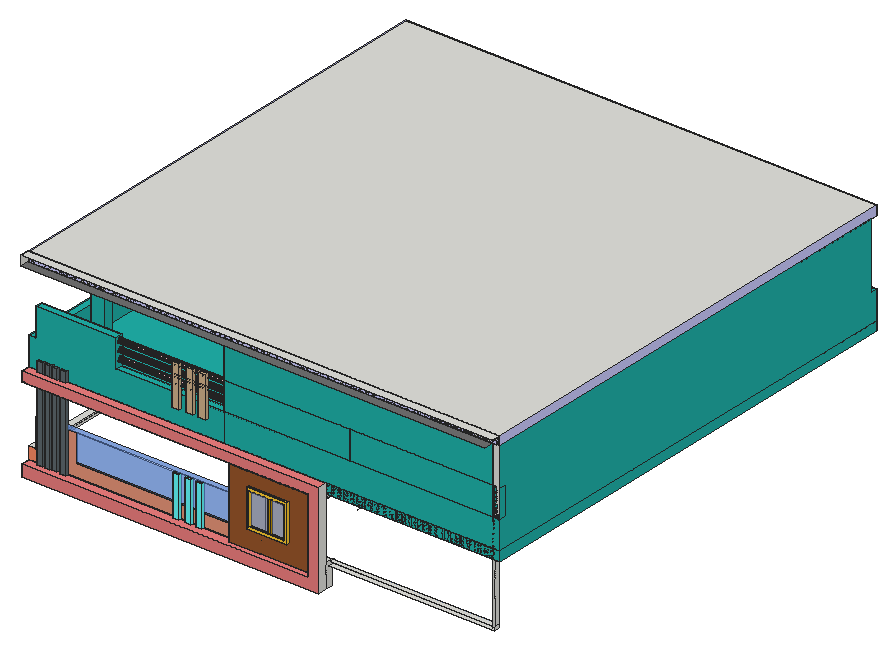
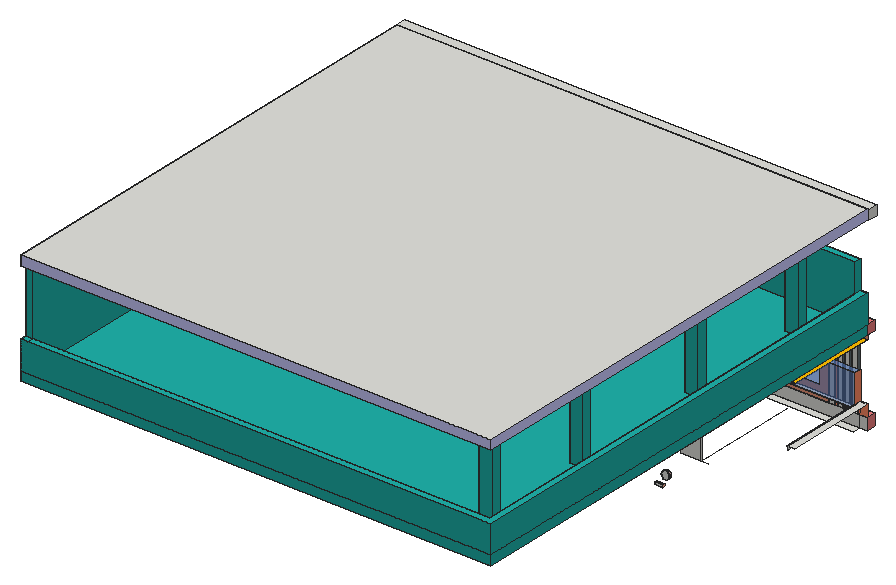
# SketchUp Ruby script. Lengths in inches.
U = 1.inch
M = Sketchup.active_model
def pt(a) = Geom::Point3d.new(a.map { |v| v * U })
def face(e, loops, mat)
  f = e.add_face(loops[0].map { |a| pt(a) })
  loops[1..].each { |l| e.add_face(l.map { |a| pt(a) }).erase! }
  f.material = f.back_material = mat if mat
  f
end
# faces: each face lists its corners as indices into pts; further lists are holes
def faces(e, pts, list, mat = nil) = list.each { |f| face(e, (f[0].is_a?(Array) ? f : [f]).map { |l| l.map { |i| pts[i] } }, mat) }
# xy, xz, yz: faces in a plane at the given z, y or x. An outline is a flat list of corners, or four numbers for a rectangle; further outlines are holes
def ring(l) = l.size == 4 ? [[l[0], l[1]], [l[2], l[1]], [l[2], l[3]], [l[0], l[3]]] : l.each_slice(2).to_a
def flat(e, list, mat, &to3) = list.each { |f| face(e, (f[0].is_a?(Array) ? f : [f]).map { |l| ring(l).map { |u, v| to3.(u, v) } }, mat) }
def xy(e, z, list, mat = nil) = flat(e, list, mat) { |x, y| [x, y, z] }
def xz(e, y, list, mat = nil) = flat(e, list, mat) { |x, z| [x, y, z] }
def yz(e, x, list, mat = nil) = flat(e, list, mat) { |y, z| [x, y, z] }
def lines(e, pts, list) = list.each { |a, b| e.add_line(pt(pts[a]), pt(pts[b])) }
# prism: a flat outline (further loops are holes) pulled along v
def prism(e, loops, v, mat = nil)
  f = face(e, loops, mat); d = Geom::Vector3d.new(v.map { |x| x * U })
  f.pushpull(f.normal.samedirection?(d) ? d.length : -d.length)
end
def box(e, o, s, mat = nil) = prism(e, [[o, [o[0] + s[0], o[1], o[2]], [o[0] + s[0], o[1] + s[1], o[2]], [o[0], o[1] + s[1], o[2]]]], [0, 0, s[2]], mat)
def at(x, y, z, deg = 0) = Geom::Transformation.translation(pt([x, y, z])) * Geom::Transformation.rotation(ORIGIN, Z_AXIS, deg.degrees)
def axes(o, x, y, z) = Geom::Transformation.new([*x, 0, *y, 0, *z, 0, *pt(o).to_a, 1])
def part(name) = M.definitions.add(name)
# library, detail: a bought-in or finely detailed component or shape, given as its bounding box
def library(name, o, s) = part(name).tap { |d| box(d.entities, o, s) }
def detail(e, o, s) = box(e.add_group.entities, o, s)
def put(e, d, t, mat = nil) = e.add_instance(d, t).tap { |i| i.material = mat if mat }
def group(e, t, mat = nil) = e.add_group.tap { |g| g.transformation = t; g.material = mat if mat }.entities
root = M.entities
M.materials.add("[0006_Pink]").color = [255, 192, 203]
M.materials.add("[0013_LightCoral]").color = [240, 128, 128]
M.materials.add("[0014_DarkSalmon]").color = [233, 150, 122]
M.materials.add("[0035_Tan]").color = [210, 180, 140]
M.materials.add("[0082_LightSeaGreen]").color = [32, 178, 170]
M.materials.add("[Color A01]").color = [255, 204, 204]
M.materials.add("[Color B02]").color = [255, 178, 153]
M.materials.add("[Color B03]").color = [255, 140, 101]
M.materials.add("[Color B07]").color = [153, 38, 0]
M.materials.add("[Color D04]").color = [255, 204, 50]
M.materials.add("[Color D05]").color = [255, 191, 0]
M.materials.add("[Color D06]").color = [204, 153, 0]
M.materials.add("[Color H03]").color = [101, 255, 255]
M.materials.add("[Color I01]").color = [204, 204, 255]
M.materials.add("[Color M05]").color = [114, 114, 114]
M.materials.add("[Formica Beige]").color = [211, 187, 149]
M.materials.add("[Formica Speckled Grey]").color = [94, 105, 111]
M.materials.add("[Translucent Glass Blue]").color = [100, 149, 237]
M.materials["[Translucent Glass Blue]"].alpha = 0.5
M.materials.add("[Translucent Glass Sky Reflection]").color = [126, 138, 183]
M.materials["[Translucent Glass Sky Reflection]"].alpha = 0.52
M.materials.add("[Translucent Glass Tinted]").color = [8, 201, 241]
M.materials["[Translucent Glass Tinted]"].alpha = 0.48
M.materials.add("[Wood Cherry Original]").color = [152, 86, 42]
xy(root,251.61,[[1.5625,0,1.5625,12,265.96,12,265.96,6,367.6875,6,367.6875,12,380.39,12,380.39,0],[265.96,6,301.8125,12],[301.8125,6,367.6875,12],[11.0625,12,380.39,21.5]])
xy(root,264.68,[[261.33,6,301.8125,12]])
xy(root,266.86,[[14.35,9,21.23,12],[23.92,9,30.79,12],[32.85,9,39.73,12],[43.48,9,50.35,12],[186.5625,9,194.61,12],
  [202.3125,9,210.36,12],[216.3125,9,224.36,12],[21.23,12,23.92,12.375],[30.79,12,32.85,12.375]])
xy(root,266.86,[[1.5625,0,367,0,367,12,224.36,12,224.36,9,216.3125,9,216.3125,12,210.36,12,210.36,9,202.3125,9,202.3125,12,194.61,12,194.61,9,186.5625,9,186.5625,12,50.35,12,50.35,9,43.48,9,43.48,12,39.73,12,39.73,9,32.85,9,32.85,12,30.79,12,30.79,9,23.92,9,23.92,12,21.23,12,21.23,9,14.35,9,14.35,12,1.5625,12]],"[0013_LightCoral]")
xy(root,267.18,[[301.8125,6,376.3125,12]])
xy(root,273.74,[[23.92,12,30.79,12.375]])
xy(root,275.45,[[61.8125,259.15,72.25,262.15]])
xy(root,277.61,[[10.5625,15.5625,10.6875,20.9375],[10.6875,15.5625,592.5625,20.9375],[10.5625,20.9375,10.6875,21],[10.6875,20.9375,592.5625,21],[10.5625,21,10.6875,127.99]])
xy(root,278.01,[[61.8125,259.15,72.25,262.15]],"[Color B02]")
xy(root,282.11,[[1.5625,12,10.5625,127.99],[10.5625,12,11.0625,127.99],[260.74,12,380.39,21],[380.39,15.5625,592.5625,21],[380.39,21,592.5625,21.5]])
xy(root,291.58,[[286.22,3,337.03,6]],"[Color D04]")
xy(root,294.58,[[311.625,5,315.25,6]])
xy(root,294.58,[[289.22,3,311.625,6],[311.625,3,315.25,5],[315.25,3,334.03,6]],"[Color D04]")
xy(root,294.68,[[181.96,262.15,184.61,265.15],[141.83,265.15,181.96,277.84],[181.96,265.15,184.61,277.84],[184.61,265.15,227.4,277.84]])
xy(root,318.07,[[186.5625,9,194.61,12]],"[Color H03]")
xy(root,318.11,[[21.23,12,32.85,12.375]])
xy(root,318.11,[[202.3125,9,210.36,12],[216.3125,9,224.36,12]],"[Color H03]")
xy(root,318.11,[[10.5625,12,21.23,12,21.23,12.375,32.85,12.375,32.85,12,260.74,12,260.74,21,10.5625,21]],"[Translucent Glass Blue]")
xy(root,324.8,[[49.5,262.15,85.5,265.15],[49.5,265.15,85.5,277.84]])
xy(root,327.74,[[181.96,262.15,184.61,265.15],[141.83,265.15,181.96,277.84],[184.61,265.15,227.4,277.84]])
xy(root,336.15,[[311.625,5,315.25,6]])
xy(root,336.15,[[289.22,3,311.625,6],[311.625,3,315.25,5],[315.25,3,334.03,6]],"[Color D04]")
xy(root,339.15,[[286.22,3,337.03,6]],"[Color D04]")
xy(root,355.61,[[1.5625,12,1.5625,127.99,10.5625,127.99,10.5625,139.1875,381.4375,139.1875,381.4375,12.02,380.39,12]],"[Color D05]")
xy(root,355.8,[[261.33,6,301.8125,12],[301.8125,6,376.3125,12],[10.5625,127.99,36.75,139.1875]])
xy(root,360.74,[[261.33,6,301.8125,12]])
xy(root,360.8,[[1.5625,12,380.39,12,381.4375,12.02,381.4375,139.1875,10.5625,139.1875,10.5625,127.99,1.5625,127.99],[380.39,12,381.4375,12,381.4375,12.02],[381.4375,12,592.5625,12,592.5625,15.5625,419.5,12.66,419.5,12.02,381.4375,12.02],[592.5625,12,601.5625,21.5],[381.4375,12.02,419.5,12.02,419.5,12.66],
  [381.4375,12.02,419.5,12.66,381.4375,12.66],[419.5,12.66,592.5625,15.5625,592.5625,265.15,36.75,265.15,36.75,139.1875,419.5,139.1875],[381.4375,12.66,419.5,139.1875],[592.5625,21.5,601.5625,21.5,601.5625,612,11.0625,612,11.0625,603,592.5625,603],[1.5625,127.99,10.5625,139.1875],
  [1.5625,139.1875,10.5625,265.15],[10.5625,139.1875,36.75,265.15],[1.5625,265.15,11.0625,265.15,11.0625,277.84,10.5625,277.84,10.5625,603,1.5625,603],[11.0625,265.15,592.5625,277.84],[10.5625,277.84,11.0625,603],
  [1.5625,603,11.0625,612]])
xy(root,360.8,[[1.5625,0,367,12]],"[0013_LightCoral]")
xy(root,360.86,[[1.5625,0,367,12]])
xy(root,361.18,[[301.8125,6,376.3125,12]])
xy(root,372.8,[[1.5625,0,380.39,12]],"[0013_LightCoral]")
xy(root,385.3,[[14.35,9,21.23,12],[23.92,9,30.79,12],[32.85,9,39.73,12],[43.48,9,50.35,12]],"[Formica Speckled Grey]")
xy(root,392.86,[[185.57,9,195.25,12],[203.38,9,213.07,12],[219.7,9,229.38,12]])
xy(root,444.8,[[249.92,12,592.5625,12.25]])
xy(root,444.93,[[203.38,9,213.07,12]],"[0035_Tan]")
xy(root,445.18,[[219.7,9,229.38,12]],"[0035_Tan]")
xy(root,445.24,[[185.57,9,195.25,12]],"[0035_Tan]")
xy(root,492.8,[[249.92,12,592.5625,12.25]])
xy(root,492.8,[[0,0,592.5625,12]],"[Color M05]")
xy(root,504.72,[[0,0,601.625,12]])
xz(root,0,[[1.5625,360.8,367,360.86]])
xz(root,0,[[1.5625,251.61,380.39,251.61,380.39,372.8,1.5625,372.8,1.5625,360.86,367,360.86,367,266.86,1.5625,266.86]],"[0013_LightCoral]")
xz(root,3,[[[286.22,291.58,337.03,339.15],[289.22,294.58,334.03,336.15]]],"[Color D04]")
xz(root,5,[[311.625,294.58,315.25,336.15]],"[Color D06]")
xz(root,6,[[[286.22,291.58,337.03,339.15],[289.22,294.58,334.03,336.15]],[311.625,294.58,315.25,336.15]])
xz(root,6,[[289.22,294.58,311.625,336.15],[315.25,294.58,334.03,336.15]],"[Translucent Glass Sky Reflection]")
xz(root,6,[[[261.33,264.68,301.8125,264.68,301.8125,267.18,376.3125,267.18,376.3125,355.8,261.33,355.8],[286.22,291.58,337.03,339.15]],[261.33,355.8,376.3125,355.8,376.3125,361.18,301.8125,361.18,301.8125,360.74,261.33,360.74]],"[Wood Cherry Original]")
xz(root,9,[[185.57,392.86,195.25,445.24],[203.38,392.86,213.07,444.93],[219.7,392.86,229.38,445.18]],"[0035_Tan]")
xz(root,9,[[186.5625,266.86,194.61,318.07],[202.3125,266.86,210.36,318.11],[216.3125,266.86,224.36,318.11]],"[Color H03]")
xz(root,9,[[14.35,266.86,21.23,385.3],[23.92,266.86,30.79,385.3],[32.85,266.86,39.73,385.3],[43.48,266.86,50.35,385.3]],"[Formica Speckled Grey]")
xz(root,12,[[1.5625,251.61,11.0625,266.86],[11.0625,251.61,265.96,251.61,265.96,264.68,261.33,264.68,261.33,266.86,11.0625,266.86],[265.96,251.61,301.8125,264.68],[301.8125,251.61,380.39,251.61,380.39,282.11,376.3125,282.11,376.3125,267.18,367,267.18,367,266.86,301.8125,266.86],[261.33,264.68,301.8125,266.86],
  [32.85,266.86,39.73,273.74],[43.48,266.86,50.35,273.74],[186.5625,266.86,194.61,283.13],[202.3125,266.86,210.36,283.13],[216.3125,266.86,224.36,283.13],
  [261.33,266.86,301.8125,282.11],[301.8125,266.86,367,267.18],[301.8125,267.18,367,282.11],[367,267.18,376.3125,282.11],[14.35,273.74,21.23,318.11],
  [23.92,273.74,30.79,318.11],[32.85,273.74,39.73,318.11],[43.48,273.74,50.35,318.11],[261.33,282.11,301.8125,355.61],[301.8125,282.11,367,355.61],
  [367,282.11,376.3125,355.61],[376.3125,282.11,380.39,355.61],[186.5625,283.13,194.61,318.07],[202.3125,283.13,210.36,318.11],[216.3125,283.13,224.36,318.11],
  [186.5625,318.07,194.61,318.11],[14.35,318.11,21.23,355.61],[23.92,318.11,30.79,355.61],[32.85,318.11,39.73,355.61],[43.48,318.11,50.35,355.61],
  [1.5625,355.61,14.35,355.8],[14.35,355.61,21.23,355.8],[21.23,355.61,23.92,355.8],[23.92,355.61,30.79,355.8],[30.79,355.61,32.85,355.8],
  [32.85,355.61,39.73,355.8],[39.73,355.61,43.48,355.8],[43.48,355.61,50.35,355.8],[50.35,355.61,261.33,355.8],[261.33,355.61,265.96,355.8],
  [265.96,355.61,301.8125,355.8],[301.8125,355.61,367,355.8],[367,355.61,376.3125,355.8],[376.3125,355.61,380.39,355.8],[14.35,355.8,21.23,360.8],
  [23.92,355.8,30.79,360.8],[32.85,355.8,39.73,360.8],[43.48,355.8,50.35,360.8],[261.33,355.8,301.8125,360.74],[301.8125,355.8,367,360.8],
  [367,355.8,376.3125,357.8],[376.3125,355.8,380.39,357.8],[367,357.8,376.3125,360.8],[376.3125,357.8,380.39,360.8],[265.96,360.74,301.8125,360.8],
  [592.5625,360.8,592.5625,372.8,594.23,372.8,594.23,444.8,592.5625,444.8,592.5625,492.8,0,492.8,0,504.72,601.5625,504.72,601.5625,360.8],[1.5625,360.8,14.35,360.86],[14.35,360.8,21.23,360.86],[21.23,360.8,23.92,360.86],[23.92,360.8,30.79,360.86],
  [30.79,360.8,32.85,360.86],[32.85,360.8,39.73,360.86],[39.73,360.8,43.48,360.86],[43.48,360.8,50.35,360.86],[376.3125,360.8,376.3125,361.18,301.8125,361.18,301.8125,360.86,50.35,360.86,50.35,372.8,380.39,372.8,380.39,360.8],
  [50.35,360.8,265.96,360.86],[265.96,360.8,301.8125,360.86],[301.8125,360.8,367,360.86],[367,360.8,376.3125,361.18],[1.5625,360.86,14.35,372.8],
  [14.35,360.86,21.23,372.8],[21.23,360.86,23.92,372.8],[23.92,360.86,30.79,372.8],[30.79,360.86,32.85,372.8],[32.85,360.86,39.73,372.8],
  [39.73,360.86,43.48,372.8],[43.48,360.86,50.35,372.8],[301.8125,360.86,367,361.18],[14.35,372.8,21.23,385.3],[23.92,372.8,30.79,385.3],
  [32.85,372.8,39.73,385.3],[43.48,372.8,50.35,385.3],[592.5625,372.8,594.23,444.8],[185.57,392.86,195.25,408.8],[203.38,392.86,213.07,408.8],
  [219.7,392.86,229.38,408.8],[185.57,408.8,195.25,444.11],[203.38,408.8,213.07,442.8],[219.7,408.8,229.38,443.36],[203.38,442.8,213.07,444.93],
  [219.7,443.36,229.38,445.18],[185.57,444.11,195.25,445.05],[185.57,445.05,195.25,445.24]])
xz(root,12,[[50.35,266.86,186.5625,266.86,186.5625,283.13,62.34,283.13,62.34,318.11,50.35,318.11],[194.61,266.86,202.3125,283.13],[210.36,266.86,216.3125,283.13],[224.36,266.86,261.33,266.86,261.33,282.11,260.74,282.11,260.74,283.13,224.36,283.13],[1.5625,355.8,14.35,360.8],
  [21.23,355.8,23.92,360.8],[30.79,355.8,32.85,360.8],[39.73,355.8,43.48,360.8],[50.35,355.8,261.33,355.8,261.33,360.74,265.96,360.74,265.96,360.8,50.35,360.8]],"[0014_DarkSalmon]")
xz(root,12,[[380.39,360.8,592.5625,372.8],[249.92,444.8,592.5625,492.8]],"[0082_LightSeaGreen]")
xz(root,12,[[1.5625,266.86,11.0625,282.11],[11.0625,266.86,14.35,266.86,14.35,318.11,10.5625,318.11,10.5625,282.11,11.0625,282.11],[21.23,266.86,23.92,318.11],[30.79,266.86,32.85,318.11],[39.73,266.86,43.48,318.11]],"[Color B03]")
xz(root,12,[[62.34,283.13,186.5625,318.11],[194.61,283.13,202.3125,318.11],[210.36,283.13,216.3125,318.11],[224.36,283.13,260.74,318.11]],"[Translucent Glass Blue]")
xz(root,12.25,[[249.92,444.8,592.5625,492.8]])
xz(root,12.375,[[21.23,266.86,21.23,318.11,32.85,318.11,32.85,266.86,30.79,266.86,30.79,273.74,23.92,273.74,23.92,266.86]])
xz(root,21,[[10.5625,277.61,10.5625,318.11,260.74,318.11,260.74,282.11,592.5625,282.11,592.5625,277.61]],"[Translucent Glass Blue]")
xz(root,127.99,[[1.5625,355.61,10.5625,355.8]])
xz(root,139.1875,[[10.5625,355.61,36.75,355.8],[36.75,355.61,381.4375,355.8],[10.5625,355.8,36.75,357.8],[36.75,355.8,381.4375,357.8],[381.4375,355.8,419.5,357.8],
  [10.5625,357.8,36.75,360.8],[36.75,357.8,381.4375,360.8],[381.4375,357.8,419.5,360.8]])
xz(root,259.15,[[59.23,285.14,60.56,285.3125,61.8,285.82,62.86,286.64,63.67,287.7,64.18,288.9375,64.36,290.26,64.18,291.59,63.67,292.82,62.86,293.89,61.8,294.7,60.56,295.21,59.23,295.39,57.91,295.21,56.67,294.7,55.61,293.89,54.79,292.82,54.28,291.59,54.11,290.26,54.28,288.9375,54.79,287.7,55.61,286.64,56.67,285.82,57.91,285.3125]],"[Color A01]")
xz(root,259.15,[[61.8125,275.45,72.25,278.01]],"[Color B02]")
xz(root,262.15,[[61.8125,275.45,72.25,278.01],[59.23,285.14,57.91,285.3125,56.67,285.82,55.61,286.64,54.79,287.7,54.28,288.9375,54.11,290.26,54.28,291.59,54.79,292.82,55.61,293.89,56.67,294.7,57.91,295.21,59.23,295.39,60.56,295.21,61.8,294.7,62.86,293.89,63.67,292.82,64.18,291.59,64.36,290.26,64.18,288.9375,63.67,287.7,62.86,286.64,61.8,285.82,60.56,285.3125]])
xz(root,262.15,[[181.96,294.68,184.61,327.74]],"[Color B07]")
xz(root,265.15,[[181.96,294.68,184.61,327.74],[10.5625,324.8,11.0625,360.8],[11.0625,324.8,36.75,360.8]])
xz(root,265.15,[[141.83,294.68,161.89,294.68,162.58,311.21,141.83,311.21],[161.89,294.68,181.96,294.68,181.96,311.21,162.58,311.21],[184.61,294.68,206,311.21],[206,294.68,227.4,311.21],[141.83,311.21,162.58,311.21,163.27,327.74,141.83,327.74],
  [162.58,311.21,181.96,311.21,181.96,327.74,163.27,327.74],[184.61,311.21,206,327.74],[206,311.21,227.4,327.74]],"[Translucent Glass Tinted]")
xz(root,277.84,[[181.96,294.68,184.61,327.74]])
yz(root,0,[[0,492.8,12,504.72]])
yz(root,1.5625,[[12,355.61,127.99,355.8],[0,360.8,12,360.86]])
yz(root,1.5625,[[0,251.61,12,266.86],[0,360.86,12,372.8]],"[0013_LightCoral]")
yz(root,10.5625,[[15.5625,277.61,21,282.11],[21,277.61,127.99,282.11],[127.99,355.61,139.1875,355.8],[127.99,355.8,139.1875,357.8],[127.99,357.8,139.1875,360.8]])
yz(root,10.5625,[[12,282.11,21,318.11]],"[Color B03]")
yz(root,14.35,[[9,266.86,12,385.3]],"[Formica Speckled Grey]")
yz(root,21.23,[[12,266.86,12.375,273.74],[12,273.74,12.375,318.11]])
yz(root,21.23,[[9,266.86,12,385.3]],"[Formica Speckled Grey]")
yz(root,23.92,[[12,266.86,12.375,273.74]])
yz(root,23.92,[[9,266.86,12,385.3]],"[Formica Speckled Grey]")
yz(root,30.79,[[12,266.86,12.375,273.74]])
yz(root,30.79,[[9,266.86,12,385.3]],"[Formica Speckled Grey]")
yz(root,32.85,[[12,266.86,12.375,273.74],[12,273.74,12.375,318.11]])
yz(root,32.85,[[9,266.86,12,385.3]],"[Formica Speckled Grey]")
yz(root,39.73,[[9,266.86,12,385.3]],"[Formica Speckled Grey]")
yz(root,43.48,[[9,266.86,12,385.3]],"[Formica Speckled Grey]")
yz(root,50.35,[[9,266.86,12,385.3]],"[Formica Speckled Grey]")
yz(root,61.8125,[[259.15,275.45,262.15,278.01]],"[Color B02]")
yz(root,72.25,[[259.15,275.45,262.15,278.01]],"[Color B02]")
yz(root,112.64,[[17.21,415.66,16.44,415.76,15.71,416.06,15.09,416.53,14.61,417.16,14.3125,417.88,14.21,418.66,14.3125,419.43,14.61,420.16,15.09,420.78,15.71,421.25,16.44,421.55,17.21,421.66,17.99,421.55,18.71,421.25,19.33,420.78,19.81,420.16,20.11,419.43,20.21,418.66,20.11,417.88,19.81,417.16,19.33,416.53,18.71,416.06,17.99,415.76],[17.21,426.28,16.44,426.38,15.71,426.68,15.09,427.16,14.61,427.78,14.3125,428.5,14.21,429.28,14.3125,430.06,14.61,430.78,15.09,431.4,15.71,431.88,16.44,432.18,17.21,432.28,17.99,432.18,18.71,431.88,19.33,431.4,19.81,430.78,20.11,430.06,20.21,429.28,20.11,428.5,19.81,427.78,19.33,427.16,18.71,426.68,17.99,426.38],[16.39,437.5,15.61,437.6,14.89,437.9,14.27,438.38,13.79,439,13.49,439.72,13.39,440.5,13.49,441.28,13.79,442,14.27,442.62,14.89,443.1,15.61,443.4,16.39,443.5,17.16,443.4,17.89,443.1,18.51,442.62,18.98,442,19.28,441.28,19.39,440.5,19.28,439.72,18.98,439,18.51,438.38,17.89,437.9,17.16,437.6]])
yz(root,141.83,[[265.15,294.68,277.84,327.74]])
yz(root,181.96,[[265.15,294.68,277.84,327.74],[262.15,311.21,265.15,327.74]])
yz(root,181.96,[[262.15,294.68,265.15,311.21]],"[Color B07]")
yz(root,184.61,[[265.15,294.68,277.84,327.74],[262.15,311.21,265.15,327.74]])
yz(root,184.61,[[262.15,294.68,265.15,311.21]],"[Color B07]")
yz(root,185.57,[[9,392.86,12,445.24]],"[0035_Tan]")
yz(root,186.5625,[[9,266.86,12,318.07]],"[Color H03]")
yz(root,194.61,[[9,266.86,12,318.07]],"[Color H03]")
yz(root,195.25,[[9,392.86,12,445.24]],"[0035_Tan]")
yz(root,202.3125,[[9,266.86,12,318.11]],"[Color H03]")
yz(root,203.38,[[9,392.86,12,444.93]],"[0035_Tan]")
yz(root,210.36,[[9,266.86,12,318.11]],"[Color H03]")
yz(root,213.07,[[9,392.86,12,444.93]],"[0035_Tan]")
yz(root,216.3125,[[9,266.86,12,318.11]],"[Color H03]")
yz(root,219.7,[[9,392.86,12,445.18]],"[0035_Tan]")
yz(root,224.36,[[9,266.86,12,318.11]],"[Color H03]")
yz(root,227.4,[[265.15,294.68,277.84,327.74]])
yz(root,229.38,[[9,392.86,12,445.18]],"[0035_Tan]")
yz(root,249.39,[[17.21,426.28,17.99,426.38,18.71,426.68,19.33,427.16,19.81,427.78,20.11,428.5,20.21,429.28,20.11,430.06,19.81,430.78,19.33,431.4,18.71,431.88,17.99,432.18,17.21,432.28,16.44,432.18,15.71,431.88,15.09,431.4,14.61,430.78,14.3125,430.06,14.21,429.28,14.3125,428.5,14.61,427.78,15.09,427.16,15.71,426.68,16.44,426.38]])
yz(root,249.76,[[17.21,415.66,17.99,415.76,18.71,416.06,19.33,416.53,19.81,417.16,20.11,417.88,20.21,418.66,20.11,419.43,19.81,420.16,19.33,420.78,18.71,421.25,17.99,421.55,17.21,421.66,16.44,421.55,15.71,421.25,15.09,420.78,14.61,420.16,14.3125,419.43,14.21,418.66,14.3125,417.88,14.61,417.16,15.09,416.53,15.71,416.06,16.44,415.76]])
yz(root,249.92,[[16.39,437.5,17.16,437.6,17.89,437.9,18.51,438.38,18.98,439,19.28,439.72,19.39,440.5,19.28,441.28,18.98,442,18.51,442.62,17.89,443.1,17.16,443.4,16.39,443.5,15.61,443.4,14.89,443.1,14.27,442.62,13.79,442,13.49,441.28,13.39,440.5,13.49,439.72,13.79,439,14.27,438.38,14.89,437.9,15.61,437.6],[12,444.8,12.25,492.8]])
yz(root,260.74,[[12,282.11,21,318.11]])
yz(root,261.33,[[6,264.68,12,355.8],[6,355.8,12,360.74]],"[Wood Cherry Original]")
yz(root,286.22,[[3,291.58,6,339.15]],"[Color D04]")
yz(root,289.22,[[3,294.58,6,336.15]],"[Color D04]")
yz(root,301.8125,[[6,264.68,12,267.18],[6,360.74,12,361.18]])
yz(root,311.625,[[5,294.58,6,336.15]],"[Color D06]")
yz(root,315.25,[[5,294.58,6,336.15]],"[Color D06]")
yz(root,334.03,[[3,294.58,6,336.15]],"[Color D04]")
yz(root,337.03,[[3,291.58,6,339.15]],"[Color D04]")
yz(root,367,[[0,360.8,12,360.86]])
yz(root,367,[[0,266.86,12,360.8]],"[0013_LightCoral]")
yz(root,376.3125,[[6,267.18,12,282.11],[6,282.11,12,355.8],[6,355.8,12,361.18]])
yz(root,380.39,[[0,251.61,12,372.8],[12,251.61,21.5,282.11]])
yz(root,381.4375,[[12.02,355.61,12.66,355.8],[12.66,355.61,139.1875,355.8],[12.02,355.8,12.66,360.8],[12.66,355.8,139.1875,360.8]])
yz(root,592.5625,[[15.5625,277.61,21,282.11],[12,282.11,15.5625,360.8],[15.5625,282.11,21,360.8],[21,282.11,21.5,360.8],[12,444.8,12.25,492.8]])
p = [[57.91,262.15,285.3125],[59.23,262.15,285.14],[59.23,259.15,285.14],[57.91,259.15,285.3125],[60.56,262.15,285.3125],[60.56,259.15,285.3125],
  [56.67,262.15,285.82],[56.67,259.15,285.82],[61.8,262.15,285.82],[61.8,259.15,285.82],[55.61,262.15,286.64],[55.61,259.15,286.64],
  [62.86,262.15,286.64],[62.86,259.15,286.64],[54.79,262.15,287.7],[54.79,259.15,287.7],[63.67,262.15,287.7],[63.67,259.15,287.7],
  [54.28,262.15,288.9375],[54.28,259.15,288.9375],[64.18,262.15,288.9375],[64.18,259.15,288.9375],[54.11,262.15,290.26],[54.11,259.15,290.26],
  [64.36,262.15,290.26],[64.36,259.15,290.26],[54.28,262.15,291.59],[54.28,259.15,291.59],[64.18,262.15,291.59],[64.18,259.15,291.59],
  [54.79,262.15,292.82],[54.79,259.15,292.82],[63.67,262.15,292.82],[63.67,259.15,292.82],[55.61,262.15,293.89],[55.61,259.15,293.89],
  [62.86,262.15,293.89],[62.86,259.15,293.89],[56.67,262.15,294.7],[56.67,259.15,294.7],[61.8,262.15,294.7],[61.8,259.15,294.7],
  [57.91,262.15,295.21],[57.91,259.15,295.21],[60.56,262.15,295.21],[60.56,259.15,295.21],[59.23,262.15,295.39],[59.23,259.15,295.39],
  [381.4375,12.02,360.8],[380.39,12,360.8],[380.39,12,357.8],[380.39,12,355.8],[380.39,12,355.61],[381.4375,12.02,355.61],
  [381.4375,12.02,355.8],[112.64,16.44,415.76],[112.64,17.21,415.66],[249.76,17.21,415.66],[249.76,16.44,415.76],[112.64,17.99,415.76],
  [249.76,17.99,415.76],[112.64,15.71,416.06],[249.76,15.71,416.06],[112.64,18.71,416.06],[249.76,18.71,416.06],[112.64,15.09,416.53],
  [249.76,15.09,416.53],[112.64,19.33,416.53],[249.76,19.33,416.53],[112.64,14.61,417.16],[249.76,14.61,417.16],[112.64,19.81,417.16],
  [249.76,19.81,417.16],[112.64,14.3125,417.88],[249.76,14.3125,417.88],[112.64,20.11,417.88],[249.76,20.11,417.88],[112.64,14.21,418.66],
  [249.76,14.21,418.66],[112.64,20.21,418.66],[249.76,20.21,418.66],[112.64,14.3125,419.43],[249.76,14.3125,419.43],[112.64,20.11,419.43],
  [249.76,20.11,419.43],[112.64,14.61,420.16],[249.76,14.61,420.16],[112.64,19.81,420.16],[249.76,19.81,420.16],[112.64,15.09,420.78],
  [249.76,15.09,420.78],[112.64,19.33,420.78],[249.76,19.33,420.78],[112.64,15.71,421.25],[249.76,15.71,421.25],[112.64,18.71,421.25],
  [249.76,18.71,421.25],[112.64,16.44,421.55],[249.76,16.44,421.55],[112.64,17.99,421.55],[249.76,17.99,421.55],[112.64,17.21,421.66],
  [249.76,17.21,421.66],[112.64,17.21,426.28],[249.39,17.21,426.28],[249.39,16.44,426.38],[112.64,16.44,426.38],[112.64,17.99,426.38],
  [249.39,17.99,426.38],[249.39,15.71,426.68],[112.64,15.71,426.68],[112.64,18.71,426.68],[249.39,18.71,426.68],[249.39,15.09,427.16],
  [112.64,15.09,427.16],[112.64,19.33,427.16],[249.39,19.33,427.16],[249.39,14.61,427.78],[112.64,14.61,427.78],[112.64,19.81,427.78],
  [249.39,19.81,427.78],[249.39,14.3125,428.5],[112.64,14.3125,428.5],[112.64,20.11,428.5],[249.39,20.11,428.5],[249.39,14.21,429.28],
  [112.64,14.21,429.28],[112.64,20.21,429.28],[249.39,20.21,429.28],[249.39,14.3125,430.06],[112.64,14.3125,430.06],[112.64,20.11,430.06],
  [249.39,20.11,430.06],[249.39,14.61,430.78],[112.64,14.61,430.78],[112.64,19.81,430.78],[249.39,19.81,430.78],[249.39,15.09,431.4],
  [112.64,15.09,431.4],[112.64,19.33,431.4],[249.39,19.33,431.4],[249.39,15.71,431.88],[112.64,15.71,431.88],[112.64,18.71,431.88],
  [249.39,18.71,431.88],[249.39,16.44,432.18],[112.64,16.44,432.18],[112.64,17.99,432.18],[249.39,17.99,432.18],[249.39,17.21,432.28],
  [112.64,17.21,432.28],[112.64,15.61,437.6],[112.64,16.39,437.5],[249.92,16.39,437.5],[249.92,15.61,437.6],[112.64,17.16,437.6],
  [249.92,17.16,437.6],[112.64,14.89,437.9],[249.92,14.89,437.9],[112.64,17.89,437.9],[249.92,17.89,437.9],[112.64,14.27,438.38],
  [249.92,14.27,438.38],[112.64,18.51,438.38],[249.92,18.51,438.38],[112.64,13.79,439],[249.92,13.79,439],[112.64,18.98,439],
  [249.92,18.98,439],[112.64,13.49,439.72],[249.92,13.49,439.72],[112.64,19.28,439.72],[249.92,19.28,439.72],[112.64,13.39,440.5],
  [249.92,13.39,440.5],[112.64,19.39,440.5],[249.92,19.39,440.5],[112.64,13.49,441.28],[249.92,13.49,441.28],[112.64,19.28,441.28],
  [249.92,19.28,441.28],[112.64,13.79,442],[249.92,13.79,442],[112.64,18.98,442],[249.92,18.98,442],[112.64,14.27,442.62],
  [249.92,14.27,442.62],[112.64,18.51,442.62],[249.92,18.51,442.62],[112.64,14.89,443.1],[249.92,14.89,443.1],[112.64,17.89,443.1],
  [249.92,17.89,443.1],[112.64,15.61,443.4],[249.92,15.61,443.4],[112.64,17.16,443.4],[249.92,17.16,443.4],[112.64,16.39,443.5],
  [249.92,16.39,443.5],[10.5625,603,324.8],[1.5625,603,324.8],[592.5625,21,408.8],[592.5625,12,408.8],[592.5625,603,408.8],
  [592.5625,612,408.8],[1.5625,127.99,357.8],[10.5625,127.99,357.8],[11.0625,127.99,324.8],[11.0625,265.15,324.8],[1.5625,265.15,324.8],
  [10.5625,265.15,324.8],[301.8125,12,282.11],[301.8125,6,282.11],[419.5,12.02,355.8],[419.5,139.1875,355.8],[381.4375,12,355.8],
  [249.92,12,372.8],[249.92,12,444.8]]
faces(root,p,[[0,1,2,3],[1,4,5,2],[6,0,3,7],[4,8,9,5],[10,6,7,11],[8,12,13,9],[14,10,11,15],[12,16,17,13],
  [18,14,15,19],[16,20,21,17],[22,18,19,23],[20,24,25,21],[26,22,23,27],[24,28,29,25],[30,26,27,31],[28,32,33,29],
  [34,30,31,35],[32,36,37,33],[38,34,35,39],[36,40,41,37],[42,38,39,43],[40,44,45,41],[46,42,43,47],[44,46,47,45]],"[Color A01]")
faces(root,p,[[48,49,50,51,52,53,54]])
faces(root,p,[[55,56,57,58],[56,59,60,57],[61,55,58,62],[59,63,64,60],[65,61,62,66],[63,67,68,64],[69,65,66,70],[67,71,72,68],
  [73,69,70,74],[71,75,76,72],[77,73,74,78],[75,79,80,76],[81,77,78,82],[79,83,84,80],[85,81,82,86],[83,87,88,84],
  [89,85,86,90],[87,91,92,88],[93,89,90,94],[91,95,96,92],[97,93,94,98],[95,99,100,96],[101,97,98,102],[99,101,102,100],
  [103,104,105,106],[107,108,104,103],[106,105,109,110],[111,112,108,107],[110,109,113,114],[115,116,112,111],[114,113,117,118],[119,120,116,115],
  [118,117,121,122],[123,124,120,119],[122,121,125,126],[127,128,124,123],[126,125,129,130],[131,132,128,127],[130,129,133,134],[135,136,132,131],
  [134,133,137,138],[139,140,136,135],[138,137,141,142],[143,144,140,139],[142,141,145,146],[147,148,144,143],[146,145,149,150],[150,149,148,147],
  [151,152,153,154],[152,155,156,153],[157,151,154,158],[155,159,160,156],[161,157,158,162],[159,163,164,160],[165,161,162,166],[163,167,168,164],
  [169,165,166,170],[167,171,172,168],[173,169,170,174],[171,175,176,172],[177,173,174,178],[175,179,180,176],[181,177,178,182],[179,183,184,180],
  [185,181,182,186],[183,187,188,184],[189,185,186,190],[187,191,192,188],[193,189,190,194],[191,195,196,192],[197,193,194,198],[195,197,198,196]],"[0006_Pink]")
lines(root,p,[[199,200],[201,202],[203,204],[205,206],[207,208],[209,210],[211,212],[213,214],[215,54],[216,217]])
g1 = group(root,at(1.5625,12,360.8),"[0082_LightSeaGreen]")
xy(g1,0,[[0,0,600,600]])
xy(g1,12,[[[0,0,600,600],[9,9,591,591]],[[9,9,591,591],[38.99,49.83,56.31,61.27],[38.99,209.65,56.31,221.08],[38.99,393.08,56.31,404.52],[38.99,537.65,56.31,549.08]],[38.99,49.83,56.31,61.27],[38.99,209.65,56.31,221.08],[38.99,393.08,56.31,404.52],
  [38.99,537.65,56.31,549.08]])
xy(g1,48,[[0,0,9,0,9,591,600,591,600,600,0,600],[111.07,0,248.36,9],[248.36,0,408.61,9],[408.61,0,591,9],[591,0,600,0,599.75,0.25,591,0.25],
  [600,0,599.75,0.25,600,0.25],[591,0.25,591,9,599.75,0.25],[599.75,0.25,591,9,600,9,600,0.25]])
xy(g1,84,[[9,0,111.07,9],[248.36,0,408.61,9],[408.61,0,600,0,600,0.25,591,0.25,591,9,408.61,9],[591,0.25,600,9]])
xy(g1,132,[[600,0,600,591,591,591,591,9],[38.99,49.83,56.31,61.27],[38.99,209.65,56.31,221.08],[38.99,393.08,56.31,404.52],[38.99,537.65,56.31,549.08]])
xz(g1,0,[[0,0,600,12],[0,12,600,12,600,48,111.07,48,111.07,84,9,84,9,48,0,48],[248.36,48,408.61,84],[408.61,48,600,84]])
xz(g1,0.25,[[591,48,600,84]])
xz(g1,9,[[9,12,9,84,111.07,84,111.07,48,591,48,591,12],[248.36,48,408.61,84],[408.61,48,591,84],[591,48,600,84]])
xz(g1,49.83,[[38.99,12,56.31,132]])
xz(g1,61.27,[[38.99,12,56.31,132]])
xz(g1,209.65,[[38.99,12,56.31,132]])
xz(g1,221.08,[[38.99,12,56.31,132]])
xz(g1,393.08,[[38.99,12,56.31,132]])
xz(g1,404.52,[[38.99,12,56.31,132]])
xz(g1,537.65,[[38.99,12,56.31,132]])
xz(g1,549.08,[[38.99,12,56.31,132]])
xz(g1,591,[[9,12,591,48],[591,48,600,132]])
xz(g1,600,[[0,0,600,12],[0,12,600,48]])
yz(g1,0,[[0,0,600,12],[0,12,600,48]])
yz(g1,9,[[9,12,591,48],[0,48,9,84]])
yz(g1,38.99,[[49.83,12,61.27,132],[209.65,12,221.08,132],[393.08,12,404.52,132],[537.65,12,549.08,132]])
yz(g1,56.31,[[49.83,12,61.27,132],[209.65,12,221.08,132],[393.08,12,404.52,132],[537.65,12,549.08,132]])
yz(g1,111.07,[[0,48,9,84]])
yz(g1,248.36,[[0,48,9,84]])
yz(g1,408.61,[[0,48,9,84]])
yz(g1,591,[[9,12,591,132],[0.25,48,9,84]])
yz(g1,600,[[0,0,600,12],[0,12,600,12,600,48,591,48,591,132,0,132,0,84,9,84,9,48,0,48],[0.25,48,9,84]])
p = [[599.75,0.25,48],[600,0,48],[600,0,84],[600,0,132],[591,9,132],[591,9,84],
  [591,9,48]]
faces(g1,p,[[0,1,2,3,4,5,6]])
g2 = group(root,at(1.5625,12,486.8))
xy(g2,0,[[174.18,211.33,320.06,232.53],[174.18,234.83,320.06,256.03],[174.18,258.33,320.06,279.53],[174.18,281.83,320.06,303.03],[174.18,305.33,320.06,326.53],
  [174.18,328.83,320.06,350.03],[174.18,352.33,320.06,373.53],[174.18,376.33,320.06,397.53],[174.18,400.33,320.06,421.53],[174.18,424.33,320.06,445.53]],"[Formica Beige]")
xy(g2,6,[[174.18,211.33,320.06,232.53],[174.18,234.83,320.06,256.03],[174.18,258.33,320.06,279.53],[174.18,281.83,320.06,303.03],[174.18,305.33,320.06,326.53],
  [174.18,328.83,320.06,350.03],[174.18,352.33,320.06,373.53],[174.18,376.33,320.06,397.53],[174.18,400.33,320.06,421.53],[174.18,424.33,320.06,445.53]])
xy(g2,6,[[[0,0,600,600],[174.18,211.33,320.06,447.36]]],"[Color I01]")
xy(g2,6,[[174.18,232.53,320.06,234.83],[174.18,256.03,320.06,258.33],[174.18,279.53,320.06,281.83],[174.18,303.03,320.06,305.33],[174.18,326.53,320.06,328.83],
  [174.18,350.03,320.06,352.33],[174.18,373.53,320.06,376.33],[174.18,397.53,320.06,400.33],[174.18,421.53,320.06,424.33],[174.18,445.53,320.06,447.36]],"[Formica Beige]")
xy(g2,8.125,[[174.18,328.83,320.06,350.03]])
xy(g2,18,[[0,0,600,600]])
xz(g2,0,[[0,6,600,18]],"[Color I01]")
xz(g2,211.33,[[174.18,0,320.06,6]],"[Formica Beige]")
xz(g2,232.53,[[174.18,0,320.06,6]],"[Formica Beige]")
xz(g2,234.83,[[174.18,0,320.06,6]],"[Formica Beige]")
xz(g2,256.03,[[174.18,0,320.06,6]],"[Formica Beige]")
xz(g2,258.33,[[174.18,0,320.06,6]],"[Formica Beige]")
xz(g2,279.53,[[174.18,0,320.06,6]],"[Formica Beige]")
xz(g2,281.83,[[174.18,0,320.06,6]],"[Formica Beige]")
xz(g2,303.03,[[174.18,0,320.06,6]],"[Formica Beige]")
xz(g2,305.33,[[174.18,0,320.06,6]],"[Formica Beige]")
xz(g2,326.53,[[174.18,0,320.06,6]],"[Formica Beige]")
xz(g2,328.83,[[174.18,6,320.06,8.125]])
xz(g2,328.83,[[174.18,0,320.06,6]],"[Formica Beige]")
xz(g2,350.03,[[174.18,6,320.06,8.125]])
xz(g2,350.03,[[174.18,0,320.06,6]],"[Formica Beige]")
xz(g2,352.33,[[174.18,0,320.06,6]],"[Formica Beige]")
xz(g2,373.53,[[174.18,0,320.06,6]],"[Formica Beige]")
xz(g2,376.33,[[174.18,0,320.06,6]],"[Formica Beige]")
xz(g2,397.53,[[174.18,0,320.06,6]],"[Formica Beige]")
xz(g2,400.33,[[174.18,0,320.06,6]],"[Formica Beige]")
xz(g2,421.53,[[174.18,0,320.06,6]],"[Formica Beige]")
xz(g2,424.33,[[174.18,0,320.06,6]],"[Formica Beige]")
xz(g2,445.53,[[174.18,0,320.06,6]],"[Formica Beige]")
xz(g2,600,[[0,6,600,18]],"[Color I01]")
yz(g2,0,[[0,6,600,18]],"[Color I01]")
yz(g2,174.18,[[328.83,6,350.03,8.125]])
yz(g2,174.18,[[211.33,0,232.53,6],[234.83,0,256.03,6],[258.33,0,279.53,6],[281.83,0,303.03,6],[305.33,0,326.53,6],
  [328.83,0,350.03,6],[352.33,0,373.53,6],[376.33,0,397.53,6],[400.33,0,421.53,6],[424.33,0,445.53,6]],"[Formica Beige]")
yz(g2,320.06,[[328.83,6,350.03,8.125]])
yz(g2,320.06,[[211.33,0,232.53,6],[234.83,0,256.03,6],[258.33,0,279.53,6],[281.83,0,303.03,6],[305.33,0,326.53,6],
  [328.83,0,350.03,6],[352.33,0,373.53,6],[376.33,0,397.53,6],[400.33,0,421.53,6],[424.33,0,445.53,6]],"[Formica Beige]")
yz(g2,600,[[0,6,600,18]],"[Color I01]")
